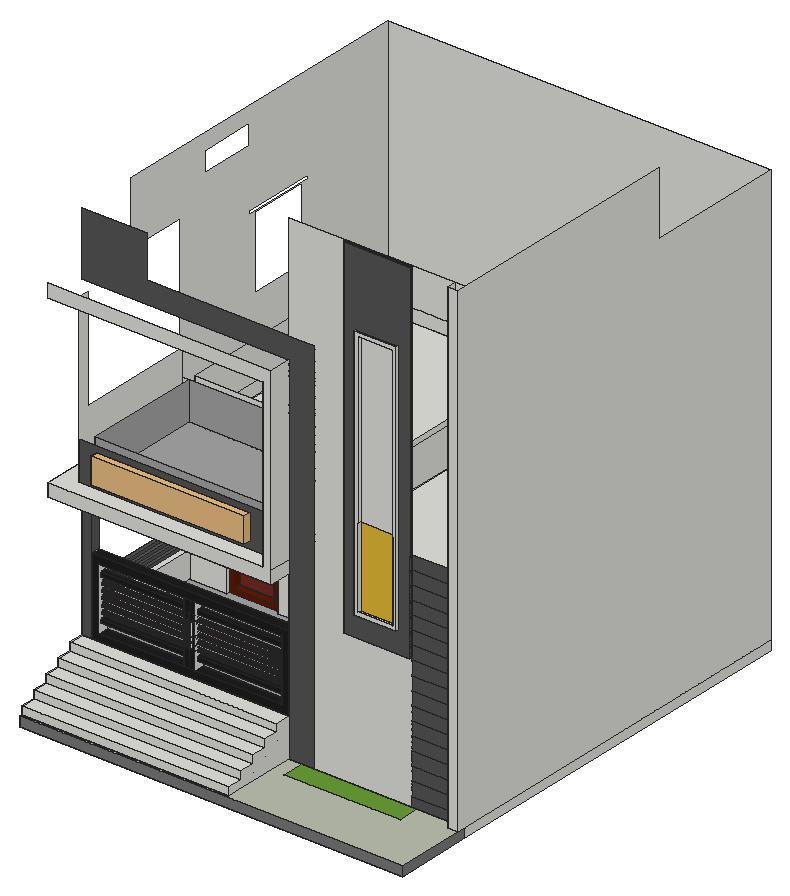
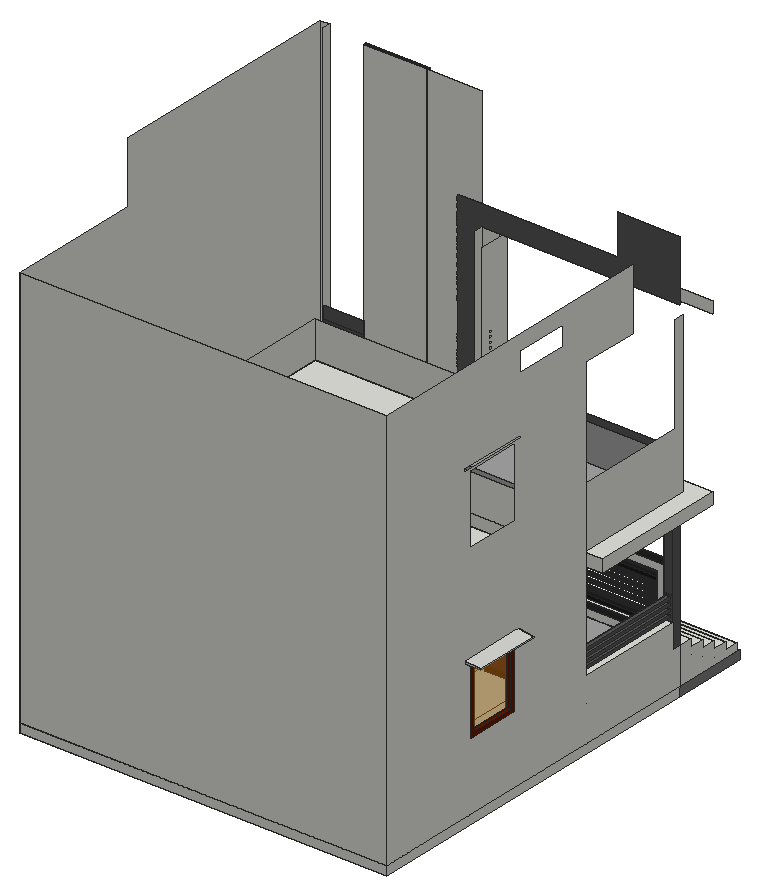
# SketchUp Ruby script. Lengths in inches.
U = 1.inch
M = Sketchup.active_model
def pt(a) = Geom::Point3d.new(a.map { |v| v * U })
def face(e, loops, mat)
  f = e.add_face(loops[0].map { |a| pt(a) })
  loops[1..].each { |l| e.add_face(l.map { |a| pt(a) }).erase! }
  f.material = f.back_material = mat if mat
  f
end
# faces: each face lists its corners as indices into pts; further lists are holes
def faces(e, pts, list, mat = nil) = list.each { |f| face(e, (f[0].is_a?(Array) ? f : [f]).map { |l| l.map { |i| pts[i] } }, mat) }
# xy, xz, yz: faces in a plane at the given z, y or x. An outline is a flat list of corners, or four numbers for a rectangle; further outlines are holes
def ring(l) = l.size == 4 ? [[l[0], l[1]], [l[2], l[1]], [l[2], l[3]], [l[0], l[3]]] : l.each_slice(2).to_a
def flat(e, list, mat, &to3) = list.each { |f| face(e, (f[0].is_a?(Array) ? f : [f]).map { |l| ring(l).map { |u, v| to3.(u, v) } }, mat) }
def xy(e, z, list, mat = nil) = flat(e, list, mat) { |x, y| [x, y, z] }
def xz(e, y, list, mat = nil) = flat(e, list, mat) { |x, z| [x, y, z] }
def yz(e, x, list, mat = nil) = flat(e, list, mat) { |y, z| [x, y, z] }
def lines(e, pts, list) = list.each { |a, b| e.add_line(pt(pts[a]), pt(pts[b])) }
# prism: a flat outline (further loops are holes) pulled along v
def prism(e, loops, v, mat = nil)
  f = face(e, loops, mat); d = Geom::Vector3d.new(v.map { |x| x * U })
  f.pushpull(f.normal.samedirection?(d) ? d.length : -d.length)
end
def box(e, o, s, mat = nil) = prism(e, [[o, [o[0] + s[0], o[1], o[2]], [o[0] + s[0], o[1] + s[1], o[2]], [o[0], o[1] + s[1], o[2]]]], [0, 0, s[2]], mat)
def at(x, y, z, deg = 0) = Geom::Transformation.translation(pt([x, y, z])) * Geom::Transformation.rotation(ORIGIN, Z_AXIS, deg.degrees)
def axes(o, x, y, z) = Geom::Transformation.new([*x, 0, *y, 0, *z, 0, *pt(o).to_a, 1])
def part(name) = M.definitions.add(name)
# library, detail: a bought-in or finely detailed component or shape, given as its bounding box
def library(name, o, s) = part(name).tap { |d| box(d.entities, o, s) }
def detail(e, o, s) = box(e.add_group.entities, o, s)
def put(e, d, t, mat = nil) = e.add_instance(d, t).tap { |i| i.material = mat if mat }
def group(e, t, mat = nil) = e.add_group.tap { |g| g.transformation = t; g.material = mat if mat }.entities
root = M.entities
M.materials.add("[Color A08]").color = [102, 0, 0]
M.materials.add("[Color B08]").color = [102, 25, 0]
M.materials.add("[Color M00]").color = [255, 255, 255]
M.materials.add("[Color M06]").color = [86, 86, 86]
M.materials.add("[Color M08]").color = [30, 30, 30]
M.materials.add("[Concrete Block Retaining Gray]").color = [121, 121, 121]
M.materials.add("[Grass Dark Green]").color = [106, 157, 55]
M.materials.add("[Mirror 02]").color = [229, 187, 54]
M.materials.add("[Pavers with Grass Brick]").color = [187, 192, 176]
M.materials.add("[Stone Vein Gray]").color = [166, 165, 165]
M.materials.add("[Translucent Glass Blue]1").color = [223, 149, 22]
M.materials["[Translucent Glass Blue]1"].alpha = 0.5
M.materials.add("[Wood Veneer 01]").color = [120, 43, 37]
c1 = part("Group\#1")
xy(c1.entities,0,[[0,0,48,6.8125]],"[Color B08]")
xy(c1.entities,4.94,[[4.94,0,43.06,6.8125]],"[Color B08]")
xy(c1.entities,79.06,[[4.94,0,43.06,6.8125]],"[Color B08]")
xy(c1.entities,84,[[0,0,48,6.8125]],"[Color B08]")
xz(c1.entities,0,[[[0,0,48,84],[4.94,4.94,43.06,79.06]]],"[Color B08]")
xz(c1.entities,6.8125,[[[0,0,48,84],[4.94,4.94,43.06,79.06]]],"[Color B08]")
xz(c1.entities,6.8125,[[4.94,4.94,43.06,79.06]],"[Wood Veneer 01]")
yz(c1.entities,0,[[0,0,6.8125,84]],"[Color B08]")
yz(c1.entities,4.94,[[0,4.94,6.8125,79.06]],"[Color B08]")
yz(c1.entities,43.06,[[0,4.94,6.8125,79.06]],"[Color B08]")
yz(c1.entities,48,[[0,0,6.8125,84]],"[Color B08]")
c2 = part("Group\#3")
xy(c2.entities,0,[[0,0,48,2.4375]],"[Color B08]")
xy(c2.entities,2.99,[[2.99,0,8.81,2.4375],[8.81,0,14.63,2.4375],[16.47,0,22.65,2.4375],[22.65,0,28.82,2.4375],[30.66,0,45.01,2.4375]],"[Color B08]")
xy(c2.entities,57.01,[[2.99,0,8.81,2.4375],[8.81,0,14.63,2.4375],[16.47,0,22.65,2.4375],[22.65,0,28.82,2.4375],[30.66,0,45.01,2.4375]],"[Color B08]")
xy(c2.entities,60,[[0,0,48,2.4375]],"[Color B08]")
xz(c2.entities,0,[[[0,0,48,60],[30.66,2.99,45.01,57.01],[16.47,2.99,28.82,57.01],[2.99,2.99,14.63,57.01]]],"[Color B08]")
xz(c2.entities,2.4375,[[[0,0,48,60],[30.66,2.99,45.01,57.01],[16.47,2.99,28.82,57.01],[2.99,2.99,14.63,57.01]]],"[Color B08]")
xz(c2.entities,2.4375,[[2.99,2.99,8.81,57.01],[8.81,2.99,14.63,57.01],[16.47,2.99,22.65,57.01],[22.65,2.99,28.82,57.01],[30.66,2.99,45.01,57.01]],"[Translucent Glass Blue]1")
yz(c2.entities,0,[[0,0,2.4375,60]],"[Color B08]")
yz(c2.entities,2.99,[[0,2.99,2.4375,57.01]],"[Color B08]")
yz(c2.entities,14.63,[[0,2.99,2.4375,57.01]],"[Color B08]")
yz(c2.entities,16.47,[[0,2.99,2.4375,57.01]],"[Color B08]")
yz(c2.entities,28.82,[[0,2.99,2.4375,57.01]],"[Color B08]")
yz(c2.entities,30.66,[[0,2.99,2.4375,57.01]],"[Color B08]")
yz(c2.entities,45.01,[[0,2.99,2.4375,57.01]],"[Color B08]")
yz(c2.entities,48,[[0,0,2.4375,60]],"[Color B08]")
c3 = part("Group\#2")
xy(c3.entities,0,[[0,0,23.0625,1.75]],"[Color B08]")
xy(c3.entities,2.13,[[2.13,0,20.93,1.75]],"[Color B08]")
xy(c3.entities,29.8,[[2.13,0,20.93,1.75]],"[Color B08]")
xy(c3.entities,31.9375,[[0,0,23.0625,1.75]],"[Color B08]")
xz(c3.entities,0,[[[0,0,23.0625,31.9375],[2.13,2.13,20.93,29.8]]],"[Color B08]")
xz(c3.entities,1.75,[[[0,0,23.0625,31.9375],[2.13,2.13,20.93,29.8]]],"[Color B08]")
xz(c3.entities,1.75,[[2.13,2.13,20.93,29.8]],"[Translucent Glass Blue]1")
yz(c3.entities,0,[[0,0,1.75,31.9375]],"[Color B08]")
yz(c3.entities,2.13,[[0,2.13,1.75,29.8]],"[Color B08]")
yz(c3.entities,20.93,[[0,2.13,1.75,29.8]],"[Color B08]")
yz(c3.entities,23.0625,[[0,0,1.75,31.9375]],"[Color B08]")
c4 = library("ENGINEER KARAN B\#1",[0.71,0,0],[427.34,23.97,4])
xy(root,0,[[16.0625,0,376.0625,73.125],[16.0625,73.125,376.0625,433.125]])
xy(root,9,[[367.0625,64.625,376.0625,73.125],[[16.0625,73.125,376.0625,433.125],[25.0625,82.125,367.0625,424.125]],[25.0625,82.125,367.0625,424.125]])
xy(root,9,[[222.91,52.375,332.28,73.125]],"[Grass Dark Green]")
xy(root,9,[[16.0625,0,376.0625,0,376.0625,64.625,367.0625,64.625,367.0625,73.125,332.28,73.125,332.28,52.375,222.91,52.375,222.91,73.125,16.0625,73.125]],"[Pavers with Grass Brick]")
xy(root,9.04,[[16.26,2.5,210.75,16.625]])
xy(root,16.24,[[16.26,2.5,210.75,16.625]])
xy(root,23.43,[[16.26,16.625,210.75,30.75]])
xy(root,30.62,[[16.26,30.75,210.75,44.875]])
xy(root,37.81,[[16.26,44.875,210.75,59]])
xy(root,45,[[16.26,59,210.75,73.125],[16.0625,73.125,25.0625,82.125],[25.0625,73.125,210.75,82.125],[25.0625,73.125,25.0625,82.125,367.0625,82.125,367.0625,294.9375,216.75,294.9375,216.75,82.125,210.75,82.125,210.75,73.125],[108.18,188.125,113.72,194.125],
  [25.0625,194.125,65.72,194.125,65.72,272.125,113.72,272.125,113.72,194.125,210.75,194.125,210.75,300.9375,367.0625,300.9375,367.0625,424.125,25.0625,424.125],[65.72,194.125,113.72,272.125]])
xy(root,45,[[25.0625,82.125,210.75,82.125,210.75,188.125,108.18,188.125,108.18,194.125,60.18,194.125,60.18,188.125,25.0625,188.125]],"[Stone Vein Gray]")
xy(root,51.82,[[31.88,73.125,112.07,82.125],[122.08,73.125,203.93,82.125]],"[Color M08]")
xy(root,59.45,[[31.88,75.08,203.93,79.9]],"[Color M08]")
xy(root,63.64,[[31.88,75.08,203.93,79.9]],"[Color M08]")
xy(root,69,[[16.0625,82.125,25.0625,188.125]])
xy(root,70.51,[[114.32,71.875,116.45,73.125],[117.64,71.875,119.76,73.125]],"[Color M00]")
xy(root,71.85,[[129.4375,188.125,177.4375,194.125]])
xy(root,72.28,[[18.56,82.125,22.8,188.0625]],"[Color M06]")
xy(root,74.9,[[18.56,82.125,22.8,188.0625]],"[Color M06]")
xy(root,75.47,[[16.0625,276.01,25.0625,331.39]])
xy(root,77.65,[[18.56,82.125,22.8,188.5]],"[Color M06]")
xy(root,80.28,[[18.56,82.125,22.8,188.5]],"[Color M06]")
xy(root,83.03,[[18.56,82.125,22.8,190]],"[Color M06]")
xy(root,85.65,[[18.56,82.125,22.8,190]],"[Color M06]")
xy(root,88.4,[[18.56,82.125,22.8,188.125]],"[Color M06]")
xy(root,91.03,[[18.56,82.125,22.8,188.125]],"[Color M06]")
xy(root,92.57,[[114.32,71.875,116.45,73.125],[117.64,71.875,119.76,73.125]],"[Color M00]")
xy(root,98.89,[[31.88,75.08,203.93,79.9]],"[Color M08]")
xy(root,103.08,[[31.88,75.08,203.93,79.9]],"[Color M08]")
xy(root,110.18,[[31.88,73.125,112.07,82.125],[122.08,73.125,203.93,82.125]],"[Color M08]")
xy(root,117,[[25.0625,73.125,210.75,82.125]],"[Color M08]")
xy(root,129,[[60.18,188.125,108.18,194.125]])
xy(root,131.85,[[129.4375,188.125,177.4375,194.125]])
xy(root,135.5,[[264.41,70.125,326.55,71.0625],[264.41,71.0625,326.55,72],[264.41,72,326.55,73.125]],"[Color M06]")
xy(root,143.66,[[16.0625,276.01,25.0625,331.39]])
xy(root,144.62,[[0.5,271.79,16.0625,336.79]])
xy(root,155.53,[[276.17,68.125,315.67,70.125],[276.17,70.125,315.67,71.0625]])
xy(root,155.53,[[276.17,71.0625,315.67,72]],"[Color M06]")
xy(root,159,[[25.0625,194.125,25.0625,424.125,367.0625,424.125,367.0625,300.9375,210.75,300.9375,210.75,194.125]])
xy(root,159.01,[[279.64,68.125,312.19,71.0625]])
xy(root,165,[[0.0625,52.25,210.75,188.125],[25.0625,194.125,210.75,194.125,210.75,300.9375,367.0625,300.9375,367.0625,424.125,25.0625,424.125]])
xy(root,165.1875,[[16.0625,73.125,25.0625,82.125]],"[Color M06]")
xy(root,171,[[216.75,82.125,367.0625,294.9375]])
xy(root,177,[[0.0625,52.25,203.0625,52.25,203.0625,67.5,17.6875,67.5,17.6875,188.125,0.0625,188.125],[17.6875,67.5,17.6875,188.125,24.85,188.125,24.85,77.25,203.0625,77.25,203.0625,67.5],[203.0625,67.5,203.8125,73.125],[203.0625,73.125,203.8125,77.25],[203.0625,77.25,210.75,82.125],
  [216.75,82.125,367.0625,294.9375]])
xy(root,177,[[24.85,77.25,24.85,188.125,210.75,188.125,210.75,82.125,203.0625,82.125,203.0625,77.25]],"[Stone Vein Gray]")
xz(root,0,[[16.0625,0,376.0625,9]],"[Concrete Block Retaining Gray]")
xz(root,2.5,[[16.26,9.04,210.75,16.24]])
xz(root,16.625,[[16.26,16.24,210.75,23.43]])
xz(root,30.75,[[16.26,23.43,210.75,30.62]])
xz(root,44.875,[[16.26,30.62,210.75,37.81]])
xz(root,52.25,[[0.0625,165,210.75,165,210.75,345,0.0625,345,0.0625,333,203.0625,333,203.0625,177,0.0625,177]])
xz(root,59,[[16.26,37.81,210.75,45]])
xz(root,64.625,[[367.0625,9,376.0625,465]])
xz(root,67.5,[[17.6875,177,203.8125,213]],"[Color M06]")
xz(root,68.125,[[[276.17,155.53,315.67,395.03],[279.64,159.01,312.19,391.56]]])
xz(root,70.125,[[[264.41,135.5,326.55,465],[276.17,155.53,315.67,395.03]]],"[Color M06]")
xz(root,71.0625,[[[276.17,155.53,315.67,395.03],[279.64,159.01,312.19,391.56]]])
xz(root,71.0625,[[[264.41,135.5,326.55,465],[276.17,155.53,315.67,395.03]]],"[Color M06]")
xz(root,71.0625,[[279.64,159.01,312.19,233.67]],"[Mirror 02]")
xz(root,71.875,[[114.32,70.51,116.45,92.57],[117.64,70.51,119.76,92.57]],"[Color M00]")
xz(root,72,[[[264.41,135.5,326.55,465],[276.17,155.53,315.67,395.03]]],"[Color M06]")
xz(root,73.125,[[16.0625,0,376.0625,9],[16.0625,9,16.26,37.81,16.26,45,16.0625,45],[16.0625,9,16.26,9,16.26,37.81],[16.26,9,210.75,37.81],[235.0625,9,326.55,9,326.55,135.5,264.41,135.5,264.41,465,210.75,465,210.75,365.8125,235.0625,365.8125],
  [16.26,37.81,210.75,45],[264.41,135.5,326.55,465]])
xz(root,73.125,[[114.32,70.51,116.45,92.57],[117.64,70.51,119.76,92.57]],"[Color M00]")
xz(root,73.125,[[210.75,9,235.0625,9,235.0625,365.8125,77.05,365.8125,77.05,405,16.0625,405,16.0625,345,210.75,345],[326.55,9,367.0625,17.85],[326.55,17.85,367.0625,30.6],[326.55,30.6,367.0625,43.35],[326.55,43.35,367.0625,56.1],
  [16.0625,45,25.0625,165.1875],[326.55,56.1,367.0625,68.85],[326.55,68.85,367.0625,81.6],[326.55,81.6,367.0625,94.35],[326.55,94.35,367.0625,107.1],
  [326.55,107.1,367.0625,119.85],[326.55,119.85,367.0625,132.6],[326.55,132.6,367.0625,145.35],[326.55,145.35,367.0625,158.1],[326.55,158.1,367.0625,170.85],
  [326.55,170.85,367.0625,183.6],[326.55,183.6,367.0625,196.35],[326.55,196.35,367.0625,209.1],[326.55,209.1,367.0625,221.85]],"[Color M06]")
xz(root,73.125,[[[25.0625,45,210.75,117],[31.88,51.82,203.93,110.18]],[112.07,51.82,117.07,51.82,116.45,66.7,116.45,70.51,114.32,70.51,114.32,92.57,116.45,92.57,116.45,87.45,117.07,110.18,112.07,110.18],[[117.07,51.82,122.08,51.82,122.08,110.18,117.07,110.18,116.45,87.45,116.45,66.7],[117.64,70.51,119.76,92.57]]],"[Color M08]")
xz(root,75.08,[[31.88,59.45,203.93,63.64],[31.88,98.89,203.93,103.08]],"[Color M08]")
xz(root,77.25,[[203.0625,177,203.8125,213]])
xz(root,77.25,[[24.85,177,203.0625,213]],"[Stone Vein Gray]")
xz(root,79.9,[[31.88,59.45,203.93,63.64],[31.88,98.89,203.93,103.08]],"[Color M08]")
xz(root,82.125,[[25.0625,9,367.0625,45],[[25.0625,45,210.75,117],[122.08,51.82,203.93,110.18],[31.88,51.82,112.07,110.18]],[216.75,45,367.0625,165],[216.75,165,367.0625,171],[216.75,171,367.0625,177],
  [216.75,177,367.0625,213]])
xz(root,82.125,[[[16.0625,69,25.0625,93],[18.56,72.28,22.8,74.9],[18.56,77.65,22.8,80.28],[18.56,83.03,22.8,85.65],[18.56,88.4,22.8,91.03]],[18.56,72.28,22.8,74.9],[18.56,77.65,22.8,80.28],[18.56,83.03,22.8,85.65],[18.56,88.4,22.8,91.03],
  [16.0625,93,25.0625,165.1875]],"[Color M06]")
xz(root,82.125,[[203.0625,177,210.75,213]],"[Stone Vein Gray]")
xz(root,188.0625,[[18.56,72.28,22.8,74.9]],"[Color M06]")
xz(root,188.125,[[[25.0625,45,60.18,45,60.18,129,108.18,129,108.18,45,210.75,45,210.75,165,16.0625,165,16.0625,69,25.0625,69],[129.4375,71.85,177.4375,131.85],[18.56,88.4,22.8,91.03]],[0.0625,165,16.0625,177],[16.0625,165,210.75,177],[16.0625,177,17.6875,213],[17.6875,177,24.85,213]])
xz(root,188.125,[[24.85,177,25.0625,213],[25.0625,177,210.75,213]],"[Stone Vein Gray]")
xz(root,188.5,[[18.56,77.65,22.8,80.28]],"[Color M06]")
xz(root,190,[[18.56,83.03,22.8,85.65]],"[Color M06]")
xz(root,194.125,[[[25.0625,45,25.0625,159,210.75,159,210.75,45,108.18,45,108.18,129,60.18,129,60.18,45],[129.4375,71.85,177.4375,131.85]],[25.0625,159,190.97,165],[190.97,159,200.91,165],[200.91,159,210.75,165],[25.0625,165,210.75,177],
  [25.0625,177,210.75,213]])
xz(root,271.79,[[0.5,144.62,16.0625,144.62,16.0625,147.68,0.5,145.35]])
xz(root,276.01,[[16.0625,75.47,25.0625,143.66]])
xz(root,294.9375,[[216.75,45,367.0625,165],[216.75,165,367.0625,171],[216.75,171,367.0625,177],[216.75,177,367.0625,213]])
xz(root,300.9375,[[210.75,45,367.0625,159],[210.75,159,367.0625,165],[210.75,165,367.0625,177],[210.75,177,367.0625,213]])
xz(root,331.39,[[16.0625,75.47,25.0625,143.66]])
xz(root,336.79,[[0.5,144.62,0.5,145.35,16.0625,147.68,16.0625,144.62]])
xz(root,424.125,[[25.0625,9,367.0625,45],[25.0625,45,367.0625,159],[25.0625,159,367.0625,165],[25.0625,165,367.0625,177],[25.0625,177,367.0625,213]])
xz(root,433.125,[[16.0625,0,376.0625,9],[16.0625,9,376.0625,405]])
yz(root,0.0625,[[52.25,165,188.125,177]])
yz(root,0.5,[[271.79,144.62,336.79,145.35]])
yz(root,16.0625,[[73.125,0,433.125,9],[[73.125,9,73.125,45,82.125,45,82.125,69,188.125,69,188.125,345,130.91,345,130.91,405,433.125,405,433.125,9],[276.01,244.22,331.39,312.41],[276.01,75.47,331.39,143.66],[216.9,371.23,269.27,390.23],[268.71,313.31,338.34,316.56],[271.79,144.62,336.79,147.68]]])
yz(root,16.0625,[[73.125,45,82.125,165.1875]],"[Color M06]")
yz(root,16.0625,[[0,0,73.125,9]],"[Concrete Block Retaining Gray]")
yz(root,16.26,[[73.125,9,16.625,9.04,2.5,9.04,2.5,16.24,16.625,16.24,16.625,23.43,30.75,23.43,30.75,30.62,44.875,30.62,44.875,37.81,59,37.81,59,45,73.125,45]])
yz(root,17.6875,[[67.5,177,67.5,333,77.25,333,77.25,237,188.125,237,188.125,177]])
yz(root,18.56,[[82.125,72.28,188.0625,74.9],[82.125,77.65,188.5,80.28],[82.125,83.03,190,85.65],[82.125,88.4,188.125,91.03]],"[Color M06]")
yz(root,22.8,[[82.125,72.28,188.0625,74.9],[82.125,77.65,188.5,80.28],[82.125,83.03,190,85.65],[82.125,88.4,188.125,91.03]],"[Color M06]")
yz(root,24.85,[[77.25,177,188.125,213]],"[Stone Vein Gray]")
yz(root,25.0625,[[73.125,45,82.125,117],[82.125,45,188.125,69],[[194.125,45,424.125,159],[276.01,75.47,331.39,143.66]],[194.125,159,424.125,165],[194.125,165,424.125,177],
  [194.125,177,424.125,213]])
yz(root,25.0625,[[73.125,117,82.125,165],[73.125,165,82.125,165.1875]],"[Color M06]")
yz(root,31.88,[[[73.125,51.82,82.125,110.18],[75.08,98.89,79.9,103.08],[75.08,59.45,79.9,63.64],[77.36,66.42,76.92,66.48,76.51,66.64,76.16,66.91,75.89,67.26,75.73,67.67,75.67,68.11,75.73,68.54,75.89,68.95,76.16,69.3,76.51,69.57,76.92,69.74,77.36,69.79,77.79,69.74,78.2,69.57,78.55,69.3,78.82,68.95,78.99,68.54,79.04,68.11,78.99,67.67,78.82,67.26,78.55,66.91,78.2,66.64,77.79,66.48],[77.36,72.67,76.92,72.73,76.51,72.89,76.16,73.16,75.89,73.51,75.73,73.92,75.67,74.36,75.73,74.79,75.89,75.2,76.16,75.55,76.51,75.82,76.92,75.99,77.36,76.04,77.79,75.99,78.2,75.82,78.55,75.55,78.82,75.2,78.99,74.79,79.04,74.36,78.99,73.92,78.82,73.51,78.55,73.16,78.2,72.89,77.79,72.73],[77.36,78.92,76.92,78.98,76.51,79.14,76.16,79.41,75.89,79.76,75.73,80.17,75.67,80.61,75.73,81.04,75.89,81.45,76.16,81.8,76.51,82.07,76.92,82.24,77.36,82.29,77.79,82.24,78.2,82.07,78.55,81.8,78.82,81.45,78.99,81.04,79.04,80.61,78.99,80.17,78.82,79.76,78.55,79.41,78.2,79.14,77.79,78.98],[77.36,85.17,76.92,85.23,76.51,85.39,76.16,85.66,75.89,86.01,75.73,86.42,75.67,86.86,75.73,87.29,75.89,87.7,76.16,88.05,76.51,88.32,76.92,88.49,77.36,88.54,77.79,88.49,78.2,88.32,78.55,88.05,78.82,87.7,78.99,87.29,79.04,86.86,78.99,86.42,78.82,86.01,78.55,85.66,78.2,85.39,77.79,85.23],[77.36,91.42,76.92,91.48,76.51,91.64,76.16,91.91,75.89,92.26,75.73,92.67,75.67,93.11,75.73,93.54,75.89,93.95,76.16,94.3,76.51,94.57,76.92,94.74,77.36,94.79,77.79,94.74,78.2,94.57,78.55,94.3,78.82,93.95,78.99,93.54,79.04,93.11,78.99,92.67,78.82,92.26,78.55,91.91,78.2,91.64,77.79,91.48],[75.74,98.89,75.73,98.92,75.67,99.36,75.73,99.79,75.89,100.2,76.16,100.55,76.51,100.82,76.92,100.99,77.36,101.04,77.79,100.99,78.2,100.82,78.55,100.55,78.82,100.2,78.99,99.79,79.04,99.36,78.99,98.92,78.97,98.89]]])
yz(root,31.88,[[77.36,66.42,76.92,66.48,76.51,66.64,76.16,66.91,75.89,67.26,75.73,67.67,75.67,68.11,75.73,68.54,75.89,68.95,76.16,69.3,76.51,69.57,76.92,69.74,77.36,69.79,77.79,69.74,78.2,69.57,78.55,69.3,78.82,68.95,78.99,68.54,79.04,68.11,78.99,67.67,78.82,67.26,78.55,66.91,78.2,66.64,77.79,66.48],[77.36,72.67,76.92,72.73,76.51,72.89,76.16,73.16,75.89,73.51,75.73,73.92,75.67,74.36,75.73,74.79,75.89,75.2,76.16,75.55,76.51,75.82,76.92,75.99,77.36,76.04,77.79,75.99,78.2,75.82,78.55,75.55,78.82,75.2,78.99,74.79,79.04,74.36,78.99,73.92,78.82,73.51,78.55,73.16,78.2,72.89,77.79,72.73],[77.36,78.92,76.92,78.98,76.51,79.14,76.16,79.41,75.89,79.76,75.73,80.17,75.67,80.61,75.73,81.04,75.89,81.45,76.16,81.8,76.51,82.07,76.92,82.24,77.36,82.29,77.79,82.24,78.2,82.07,78.55,81.8,78.82,81.45,78.99,81.04,79.04,80.61,78.99,80.17,78.82,79.76,78.55,79.41,78.2,79.14,77.79,78.98],[77.36,85.17,76.92,85.23,76.51,85.39,76.16,85.66,75.89,86.01,75.73,86.42,75.67,86.86,75.73,87.29,75.89,87.7,76.16,88.05,76.51,88.32,76.92,88.49,77.36,88.54,77.79,88.49,78.2,88.32,78.55,88.05,78.82,87.7,78.99,87.29,79.04,86.86,78.99,86.42,78.82,86.01,78.55,85.66,78.2,85.39,77.79,85.23],[77.36,91.42,76.92,91.48,76.51,91.64,76.16,91.91,75.89,92.26,75.73,92.67,75.67,93.11,75.73,93.54,75.89,93.95,76.16,94.3,76.51,94.57,76.92,94.74,77.36,94.79,77.79,94.74,78.2,94.57,78.55,94.3,78.82,93.95,78.99,93.54,79.04,93.11,78.99,92.67,78.82,92.26,78.55,91.91,78.2,91.64,77.79,91.48]],"[Color A08]")
yz(root,31.88,[[75.08,59.45,79.9,63.64],[75.08,98.89,75.08,103.08,79.9,103.08,79.9,98.89,78.97,98.89,78.99,98.92,79.04,99.36,78.99,99.79,78.82,100.2,78.55,100.55,78.2,100.82,77.79,100.99,77.36,101.04,76.92,100.99,76.51,100.82,76.16,100.55,75.89,100.2,75.73,99.79,75.67,99.36,75.73,98.92,75.74,98.89],[75.74,98.89,78.97,98.89,78.99,98.92,79.04,99.36,78.99,99.79,78.82,100.2,78.55,100.55,78.2,100.82,77.79,100.99,77.36,101.04,76.92,100.99,76.51,100.82,76.16,100.55,75.89,100.2,75.73,99.79,75.67,99.36,75.73,98.92]],"[Color M08]")
yz(root,60.18,[[188.125,45,194.125,129]])
yz(root,108.18,[[188.125,45,194.125,129]])
yz(root,112.07,[[73.125,51.82,82.125,110.18]],"[Color M08]")
yz(root,114.32,[[71.875,70.51,73.125,92.57]],"[Color M00]")
yz(root,116.45,[[71.875,70.51,73.125,92.57]],"[Color M00]")
yz(root,117.64,[[71.875,70.51,73.125,92.57]],"[Color M00]")
yz(root,119.76,[[71.875,70.51,73.125,92.57]],"[Color M00]")
yz(root,122.08,[[73.125,51.82,82.125,110.18]])
yz(root,129.4375,[[188.125,71.85,194.125,131.85]])
yz(root,177.4375,[[188.125,71.85,194.125,131.85]])
yz(root,203.0625,[[[52.25,177,52.25,333,82.125,333,82.125,213,77.25,213,77.25,177],[70.38,239.52,74.13,242.52],[70.38,244.4,74.13,247.4],[70.38,249.27,74.13,252.27],[70.38,254.15,74.13,257.15]]])
yz(root,203.0625,[[77.25,177,82.125,213]],"[Stone Vein Gray]")
yz(root,203.63,[[77.36,78.92,77.79,78.98,78.2,79.14,78.55,79.41,78.82,79.76,78.99,80.17,79.04,80.61,78.99,81.04,78.82,81.45,78.55,81.8,78.2,82.07,77.79,82.24,77.36,82.29,76.92,82.24,76.51,82.07,76.16,81.8,75.89,81.45,75.73,81.04,75.67,80.61,75.73,80.17,75.89,79.76,76.16,79.41,76.51,79.14,76.92,78.98]],"[Color A08]")
yz(root,203.8125,[[67.5,177,77.25,237]])
yz(root,203.93,[[[73.125,51.82,82.125,110.18],[75.08,98.89,79.9,103.08],[75.08,59.45,79.9,63.64],[77.36,91.42,77.79,91.48,78.2,91.64,78.55,91.91,78.82,92.26,78.99,92.67,79.04,93.11,78.99,93.54,78.82,93.95,78.55,94.3,78.2,94.57,77.79,94.74,77.36,94.79,76.92,94.74,76.51,94.57,76.16,94.3,75.89,93.95,75.73,93.54,75.67,93.11,75.73,92.67,75.89,92.26,76.16,91.91,76.51,91.64,76.92,91.48],[77.36,85.17,77.79,85.23,78.2,85.39,78.55,85.66,78.82,86.01,78.99,86.42,79.04,86.86,78.99,87.29,78.82,87.7,78.55,88.05,78.2,88.32,77.79,88.49,77.36,88.54,76.92,88.49,76.51,88.32,76.16,88.05,75.89,87.7,75.73,87.29,75.67,86.86,75.73,86.42,75.89,86.01,76.16,85.66,76.51,85.39,76.92,85.23]]],"[Color M08]")
yz(root,206.07,[[77.36,72.67,77.79,72.73,78.2,72.89,78.55,73.16,78.82,73.51,78.99,73.92,79.04,74.36,78.99,74.79,78.82,75.2,78.55,75.55,78.2,75.82,77.79,75.99,77.36,76.04,76.92,75.99,76.51,75.82,76.16,75.55,75.89,75.2,75.73,74.79,75.67,74.36,75.73,73.92,75.89,73.51,76.16,73.16,76.51,72.89,76.92,72.73]],"[Color A08]")
yz(root,206.13,[[77.36,66.42,77.79,66.48,78.2,66.64,78.55,66.91,78.82,67.26,78.99,67.67,79.04,68.11,78.99,68.54,78.82,68.95,78.55,69.3,78.2,69.57,77.79,69.74,77.36,69.79,76.92,69.74,76.51,69.57,76.16,69.3,75.89,68.95,75.73,68.54,75.67,68.11,75.73,67.67,75.89,67.26,76.16,66.91,76.51,66.64,76.92,66.48]],"[Color A08]")
yz(root,210.75,[[73.125,9,73.125,45,59,45,59,37.81,44.875,37.81,44.875,30.62,30.75,30.62,30.75,23.43,16.625,23.43,16.625,16.24,2.5,16.24,2.5,9.04,16.625,9.04],[73.125,45,82.125,117],[82.125,45,188.125,165],[194.125,45,300.9375,159],[73.125,117,82.125,165],
  [194.125,159,300.9375,165],[52.25,165,73.125,177],[73.125,165,188.125,177],[194.125,165,300.9375,177],[52.25,177,73.125,345],
  [73.125,177,82.125,345],[194.125,177,300.9375,213]])
yz(root,210.75,[[82.125,177,188.125,213]],"[Stone Vein Gray]")
yz(root,216.75,[[82.125,45,294.9375,165],[82.125,165,294.9375,171],[82.125,171,164.89,177],[164.89,171,176.14,177],[176.14,171,294.9375,177],
  [82.125,177,294.9375,213]])
yz(root,264.41,[[70.125,135.5,71.0625,465],[71.0625,135.5,72,465],[72,135.5,73.125,465]],"[Color M06]")
yz(root,276.17,[[68.125,155.53,70.125,395.03],[70.125,155.53,71.0625,395.03]])
yz(root,276.17,[[71.0625,155.53,72,395.03]],"[Color M06]")
yz(root,279.64,[[68.125,159.01,71.0625,233.67]])
yz(root,312.19,[[68.125,159.01,71.0625,233.67]])
yz(root,315.67,[[68.125,155.53,70.125,395.03],[70.125,155.53,71.0625,395.03]])
yz(root,315.67,[[71.0625,155.53,72,395.03]],"[Color M06]")
yz(root,326.55,[[72,135.5,73.125,145.35],[72,145.35,73.125,158.1],[72,158.1,73.125,170.85],[72,170.85,73.125,183.6],[72,183.6,73.125,196.35],
  [72,196.35,73.125,209.1],[72,209.1,73.125,221.85]])
yz(root,326.55,[[70.125,135.5,71.0625,145.35],[71.0625,135.5,72,145.35],[70.125,145.35,71.0625,158.1],[71.0625,145.35,72,158.1],[70.125,158.1,71.0625,170.85],
  [71.0625,158.1,72,170.85],[70.125,170.85,71.0625,183.6],[71.0625,170.85,72,183.6],[70.125,183.6,71.0625,196.35],[71.0625,183.6,72,196.35],
  [70.125,196.35,71.0625,209.1],[71.0625,196.35,72,209.1],[70.125,209.1,71.0625,221.85],[71.0625,209.1,72,221.85]],"[Color M06]")
yz(root,367.0625,[[64.625,9,73.125,465],[82.125,45,294.9375,165],[300.9375,45,424.125,159],[300.9375,159,424.125,165],[82.125,165,294.9375,171],
  [300.9375,165,424.125,177],[82.125,171,294.9375,177],[82.125,177,294.9375,213],[300.9375,177,424.125,213]])
yz(root,376.0625,[[73.125,0,433.125,9],[64.625,9,433.125,9,433.125,405,300.9375,405,300.9375,465,64.625,465]])
yz(root,376.0625,[[0,0,73.125,9]],"[Concrete Block Retaining Gray]")
p = [[210.75,16.625,9.04],[16.26,16.625,9.04],[16.26,73.125,9],[210.75,73.125,9],[31.88,76.92,66.48],[31.88,77.36,66.42],
  [206.13,77.36,66.42],[206.13,76.92,66.48],[31.88,77.79,66.48],[206.13,77.79,66.48],[31.88,76.51,66.64],[206.13,76.51,66.64],
  [31.88,78.2,66.64],[206.13,78.2,66.64],[31.88,76.16,66.91],[206.13,76.16,66.91],[31.88,78.55,66.91],[206.13,78.55,66.91],
  [31.88,75.89,67.26],[206.13,75.89,67.26],[31.88,78.82,67.26],[206.13,78.82,67.26],[31.88,75.73,67.67],[206.13,75.73,67.67],
  [31.88,78.99,67.67],[206.13,78.99,67.67],[31.88,75.67,68.11],[206.13,75.67,68.11],[31.88,79.04,68.11],[206.13,79.04,68.11],
  [31.88,75.73,68.54],[206.13,75.73,68.54],[31.88,78.99,68.54],[206.13,78.99,68.54],[31.88,75.89,68.95],[206.13,75.89,68.95],
  [31.88,78.82,68.95],[206.13,78.82,68.95],[31.88,76.16,69.3],[206.13,76.16,69.3],[31.88,78.55,69.3],[206.13,78.55,69.3],
  [31.88,76.51,69.57],[206.13,76.51,69.57],[31.88,78.2,69.57],[206.13,78.2,69.57],[31.88,76.92,69.74],[206.13,76.92,69.74],
  [31.88,77.79,69.74],[206.13,77.79,69.74],[31.88,77.36,69.79],[206.13,77.36,69.79],[31.88,76.51,72.89],[31.88,76.92,72.73],
  [206.07,76.92,72.73],[206.07,76.51,72.89],[31.88,77.36,72.67],[206.07,77.36,72.67],[31.88,77.79,72.73],[206.07,77.79,72.73],
  [31.88,78.2,72.89],[206.07,78.2,72.89],[31.88,76.16,73.16],[206.07,76.16,73.16],[31.88,78.55,73.16],[206.07,78.55,73.16],
  [31.88,75.89,73.51],[206.07,75.89,73.51],[31.88,78.82,73.51],[206.07,78.82,73.51],[31.88,75.73,73.92],[206.07,75.73,73.92],
  [31.88,78.99,73.92],[206.07,78.99,73.92],[31.88,75.67,74.36],[206.07,75.67,74.36],[31.88,79.04,74.36],[206.07,79.04,74.36],
  [31.88,75.73,74.79],[206.07,75.73,74.79],[31.88,78.99,74.79],[206.07,78.99,74.79],[31.88,75.89,75.2],[206.07,75.89,75.2],
  [31.88,78.82,75.2],[206.07,78.82,75.2],[31.88,76.16,75.55],[206.07,76.16,75.55],[31.88,78.55,75.55],[206.07,78.55,75.55],
  [31.88,76.51,75.82],[206.07,76.51,75.82],[31.88,78.2,75.82],[206.07,78.2,75.82],[31.88,76.92,75.99],[206.07,76.92,75.99],
  [31.88,77.79,75.99],[206.07,77.79,75.99],[31.88,77.36,76.04],[206.07,77.36,76.04],[31.88,76.92,78.98],[31.88,77.36,78.92],
  [203.63,77.36,78.92],[203.63,76.92,78.98],[31.88,77.79,78.98],[203.63,77.79,78.98],[31.88,76.51,79.14],[203.63,76.51,79.14],
  [31.88,78.2,79.14],[203.63,78.2,79.14],[31.88,76.16,79.41],[203.63,76.16,79.41],[31.88,78.55,79.41],[203.63,78.55,79.41],
  [31.88,75.89,79.76],[203.63,75.89,79.76],[31.88,78.82,79.76],[203.63,78.82,79.76],[31.88,75.73,80.17],[203.63,75.73,80.17],
  [31.88,78.99,80.17],[203.63,78.99,80.17],[31.88,75.67,80.61],[203.63,75.67,80.61],[31.88,79.04,80.61],[203.63,79.04,80.61],
  [31.88,75.73,81.04],[203.63,75.73,81.04],[31.88,78.99,81.04],[203.63,78.99,81.04],[31.88,75.89,81.45],[203.63,75.89,81.45],
  [31.88,78.82,81.45],[203.63,78.82,81.45],[31.88,76.16,81.8],[203.63,76.16,81.8],[31.88,78.55,81.8],[203.63,78.55,81.8],
  [31.88,76.51,82.07],[203.63,76.51,82.07],[31.88,78.2,82.07],[203.63,78.2,82.07],[31.88,76.92,82.24],[203.63,76.92,82.24],
  [31.88,77.79,82.24],[203.63,77.79,82.24],[31.88,77.36,82.29],[203.63,77.36,82.29],[31.88,76.51,85.39],[31.88,76.92,85.23],
  [203.93,76.92,85.23],[203.93,76.51,85.39],[31.88,77.36,85.17],[203.93,77.36,85.17],[31.88,77.79,85.23],[203.93,77.79,85.23],
  [31.88,78.2,85.39],[203.93,78.2,85.39],[31.88,76.16,85.66],[203.93,76.16,85.66],[31.88,78.55,85.66],[203.93,78.55,85.66],
  [31.88,75.89,86.01],[203.93,75.89,86.01],[31.88,78.82,86.01],[203.93,78.82,86.01],[31.88,75.73,86.42],[203.93,75.73,86.42],
  [31.88,78.99,86.42],[203.93,78.99,86.42],[31.88,75.67,86.86],[203.93,75.67,86.86],[31.88,79.04,86.86],[203.93,79.04,86.86],
  [31.88,75.73,87.29],[203.93,75.73,87.29],[31.88,78.99,87.29],[203.93,78.99,87.29],[31.88,75.89,87.7],[203.93,75.89,87.7],
  [31.88,78.82,87.7],[203.93,78.82,87.7],[31.88,76.16,88.05],[203.93,76.16,88.05],[31.88,78.55,88.05],[203.93,78.55,88.05],
  [31.88,76.51,88.32],[203.93,76.51,88.32],[31.88,78.2,88.32],[203.93,78.2,88.32],[31.88,76.92,88.49],[203.93,76.92,88.49],
  [31.88,77.79,88.49],[203.93,77.79,88.49],[31.88,77.36,88.54],[203.93,77.36,88.54],[31.88,76.92,91.48],[31.88,77.36,91.42],
  [203.93,77.36,91.42],[203.93,76.92,91.48],[31.88,77.79,91.48],[203.93,77.79,91.48],[31.88,76.51,91.64],[203.93,76.51,91.64],
  [31.88,78.2,91.64],[203.93,78.2,91.64],[31.88,76.16,91.91],[203.93,76.16,91.91],[31.88,78.55,91.91],[203.93,78.55,91.91],
  [31.88,75.89,92.26],[203.93,75.89,92.26],[31.88,78.82,92.26],[203.93,78.82,92.26],[31.88,75.73,92.67],[203.93,75.73,92.67],
  [31.88,78.99,92.67],[203.93,78.99,92.67],[31.88,75.67,93.11],[203.93,75.67,93.11],[31.88,79.04,93.11],[203.93,79.04,93.11],
  [31.88,75.73,93.54],[203.93,75.73,93.54],[31.88,78.99,93.54],[203.93,78.99,93.54],[31.88,75.89,93.95],[203.93,75.89,93.95],
  [31.88,78.82,93.95],[203.93,78.82,93.95],[31.88,76.16,94.3],[203.93,76.16,94.3],[31.88,78.55,94.3],[203.93,78.55,94.3],
  [31.88,76.51,94.57],[203.93,76.51,94.57],[31.88,78.2,94.57],[203.93,78.2,94.57],[31.88,76.92,94.74],[203.93,76.92,94.74],
  [31.88,77.79,94.74],[203.93,77.79,94.74],[31.88,77.36,94.79],[203.93,77.36,94.79],[0.5,271.79,145.35],[16.0625,271.79,147.68],
  [16.0625,336.79,147.68],[0.5,336.79,145.35],[25.0625,188.125,45],[16.0625,188.125,45],[326.55,73.125,5.1],[367.0625,73.125,5.1],
  [16.26,30.75,16.24],[210.75,30.75,16.24],[16.26,44.875,23.43],[210.75,44.875,23.43],[16.26,59,30.62],[210.75,59,30.62]]
faces(root,p,[[0,1,2,3],[244,245,246,247]])
faces(root,p,[[4,5,6,7],[5,8,9,6],[10,4,7,11],[8,12,13,9],[14,10,11,15],[12,16,17,13],[18,14,15,19],[16,20,21,17],
  [22,18,19,23],[20,24,25,21],[26,22,23,27],[24,28,29,25],[30,26,27,31],[28,32,33,29],[34,30,31,35],[32,36,37,33],
  [38,34,35,39],[36,40,41,37],[42,38,39,43],[40,44,45,41],[46,42,43,47],[44,48,49,45],[50,46,47,51],[48,50,51,49],
  [52,53,54,55],[53,56,57,54],[56,58,59,57],[58,60,61,59],[62,52,55,63],[60,64,65,61],[66,62,63,67],[64,68,69,65],
  [70,66,67,71],[68,72,73,69],[74,70,71,75],[72,76,77,73],[78,74,75,79],[76,80,81,77],[82,78,79,83],[80,84,85,81],
  [86,82,83,87],[84,88,89,85],[90,86,87,91],[88,92,93,89],[94,90,91,95],[92,96,97,93],[98,94,95,99],[96,98,99,97],
  [100,101,102,103],[101,104,105,102],[106,100,103,107],[104,108,109,105],[110,106,107,111],[108,112,113,109],[114,110,111,115],[112,116,117,113],
  [118,114,115,119],[116,120,121,117],[122,118,119,123],[120,124,125,121],[126,122,123,127],[124,128,129,125],[130,126,127,131],[128,132,133,129],
  [134,130,131,135],[132,136,137,133],[138,134,135,139],[136,140,141,137],[142,138,139,143],[140,144,145,141],[146,142,143,147],[144,146,147,145],
  [148,149,150,151],[149,152,153,150],[152,154,155,153],[154,156,157,155],[158,148,151,159],[156,160,161,157],[162,158,159,163],[160,164,165,161],
  [166,162,163,167],[164,168,169,165],[170,166,167,171],[168,172,173,169],[174,170,171,175],[172,176,177,173],[178,174,175,179],[176,180,181,177],
  [182,178,179,183],[180,184,185,181],[186,182,183,187],[184,188,189,185],[190,186,187,191],[188,192,193,189],[194,190,191,195],[192,194,195,193],
  [196,197,198,199],[197,200,201,198],[202,196,199,203],[200,204,205,201],[206,202,203,207],[204,208,209,205],[210,206,207,211],[208,212,213,209],
  [214,210,211,215],[212,216,217,213],[218,214,215,219],[216,220,221,217],[222,218,219,223],[220,224,225,221],[226,222,223,227],[224,228,229,225],
  [230,226,227,231],[228,232,233,229],[234,230,231,235],[232,236,237,233],[238,234,235,239],[236,240,241,237],[242,238,239,243],[240,242,243,241]],"[Color A08]")
lines(root,p,[[248,249],[250,251],[252,253],[254,255],[256,257]])
put(root,c1,at(60.18,190.125,45))
put(root,c2,at(129.4375,188.125,71.85))
put(root,c3,axes([16.0625,331.39,75.47],[0,-2.40108,0],[2,0,0],[0,0,2.13503]))
put(root,c4,axes([34.16,67.5,183.65],[0.336,0,0],[0,0,1],[0,-1.68,0]))
